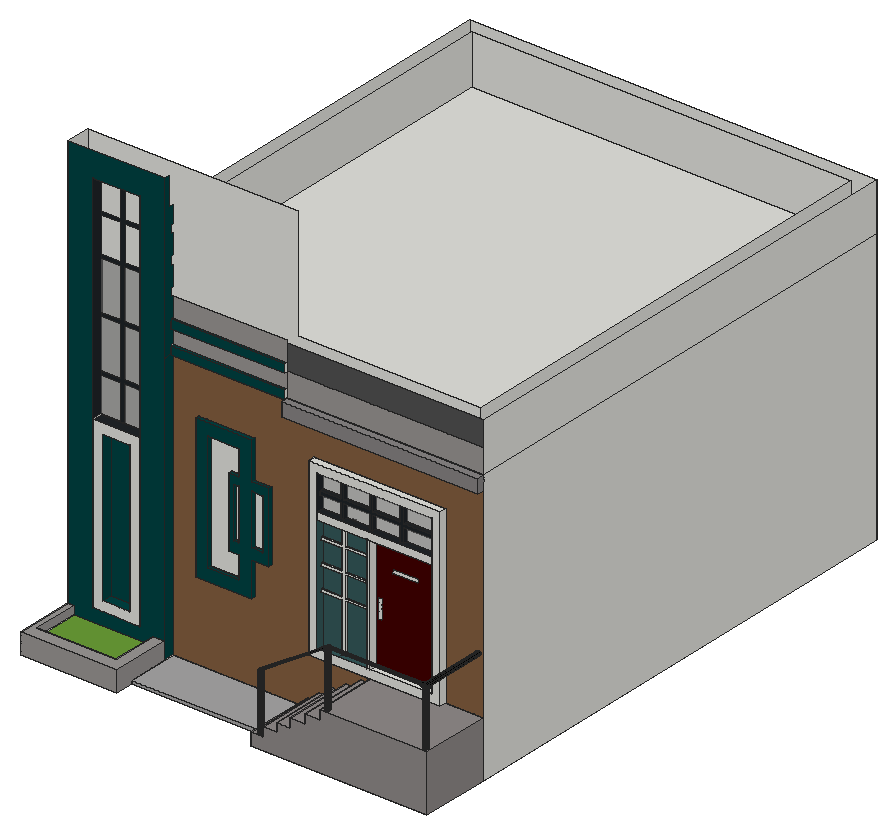
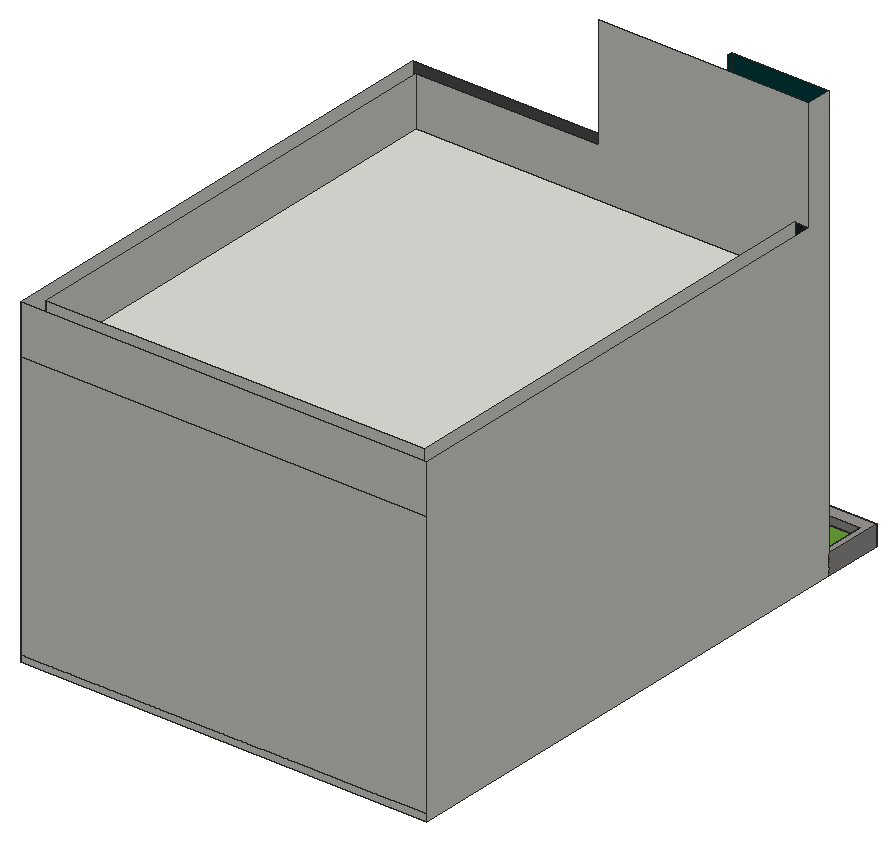
# SketchUp Ruby script. Lengths in inches.
U = 1.inch
M = Sketchup.active_model
def pt(a) = Geom::Point3d.new(a.map { |v| v * U })
def face(e, loops, mat)
  f = e.add_face(loops[0].map { |a| pt(a) })
  loops[1..].each { |l| e.add_face(l.map { |a| pt(a) }).erase! }
  f.material = f.back_material = mat if mat
  f
end
# faces: each face lists its corners as indices into pts; further lists are holes
def faces(e, pts, list, mat = nil) = list.each { |f| face(e, (f[0].is_a?(Array) ? f : [f]).map { |l| l.map { |i| pts[i] } }, mat) }
# xy, xz, yz: faces in a plane at the given z, y or x. An outline is a flat list of corners, or four numbers for a rectangle; further outlines are holes
def ring(l) = l.size == 4 ? [[l[0], l[1]], [l[2], l[1]], [l[2], l[3]], [l[0], l[3]]] : l.each_slice(2).to_a
def flat(e, list, mat, &to3) = list.each { |f| face(e, (f[0].is_a?(Array) ? f : [f]).map { |l| ring(l).map { |u, v| to3.(u, v) } }, mat) }
def xy(e, z, list, mat = nil) = flat(e, list, mat) { |x, y| [x, y, z] }
def xz(e, y, list, mat = nil) = flat(e, list, mat) { |x, z| [x, y, z] }
def yz(e, x, list, mat = nil) = flat(e, list, mat) { |y, z| [x, y, z] }
def lines(e, pts, list) = list.each { |a, b| e.add_line(pt(pts[a]), pt(pts[b])) }
# prism: a flat outline (further loops are holes) pulled along v
def prism(e, loops, v, mat = nil)
  f = face(e, loops, mat); d = Geom::Vector3d.new(v.map { |x| x * U })
  f.pushpull(f.normal.samedirection?(d) ? d.length : -d.length)
end
def box(e, o, s, mat = nil) = prism(e, [[o, [o[0] + s[0], o[1], o[2]], [o[0] + s[0], o[1] + s[1], o[2]], [o[0], o[1] + s[1], o[2]]]], [0, 0, s[2]], mat)
def at(x, y, z, deg = 0) = Geom::Transformation.translation(pt([x, y, z])) * Geom::Transformation.rotation(ORIGIN, Z_AXIS, deg.degrees)
def axes(o, x, y, z) = Geom::Transformation.new([*x, 0, *y, 0, *z, 0, *pt(o).to_a, 1])
def part(name) = M.definitions.add(name)
# library, detail: a bought-in or finely detailed component or shape, given as its bounding box
def library(name, o, s) = part(name).tap { |d| box(d.entities, o, s) }
def detail(e, o, s) = box(e.add_group.entities, o, s)
def put(e, d, t, mat = nil) = e.add_instance(d, t).tap { |i| i.material = mat if mat }
def group(e, t, mat = nil) = e.add_group.tap { |g| g.transformation = t; g.material = mat if mat }.entities
root = M.entities
M.materials.add("[0022_Maroon]").color = [66, 0, 0]
M.materials.add("[0079_Teal]").color = [0, 66, 66]
M.materials.add("[0081_CadetBlue]1").color = [52, 88, 89]
M.materials.add("[0099_LightSteelBlue]").color = [32, 36, 40]
M.materials.add("[0137_Black]").color = [0, 0, 0]
M.materials.add("[Brick Antique 01]").color = [132, 94, 64]
M.materials.add("[Brick Tumbled]").color = [135, 132, 132]
M.materials.add("[Concrete Aggregate Smoke]").color = [154, 150, 148]
M.materials.add("[Grass Dark Green]").color = [106, 157, 55]
M.materials.add("[Sketchy Scales]").color = [81, 81, 81]
M.materials.add("[Stone Marble]").color = [143, 138, 136]
M.materials.add("[Stone Vein Gray]").color = [166, 165, 165]
M.materials.add("[Translucent Glass Gray]").color = [128, 128, 128]
M.materials["[Translucent Glass Gray]"].alpha = 0.5
xy(root,0,[[0,0,0,51,5.305,51,5.305,11.375,72.805,11.375,72.805,51,82.708,51,82.708,0],[197.432,0,348,60],[5.305,11.375,72.805,51],[82.708,15.477,197.432,60],[0,51,82.708,60],
  [0,60,348,480]])
xy(root,3,[[82.708,15.477,197.432,60]],"[Stone Vein Gray]")
xy(root,10.4,[[202.157,1.901,201.64,1.969,201.157,2.169,200.743,2.487,200.425,2.901,200.225,3.383,200.157,3.901,200.225,4.419,200.425,4.901,200.743,5.315,201.157,5.633,201.64,5.833,202.157,5.901,202.675,5.833,203.157,5.633,203.571,5.315,203.889,4.901,204.089,4.419,204.157,3.901,204.089,3.383,203.889,2.901,203.571,2.487,203.157,2.169,202.675,1.969]],"[0137_Black]")
xy(root,10.4,[[[197.432,0,207.495,60],[202.157,1.901,201.64,1.969,201.157,2.169,200.743,2.487,200.425,2.901,200.225,3.383,200.157,3.901,200.225,4.419,200.425,4.901,200.743,5.315,201.157,5.633,201.64,5.833,202.157,5.901,202.675,5.833,203.157,5.633,203.571,5.315,203.889,4.901,204.089,4.419,204.157,3.901,204.089,3.383,203.889,2.901,203.571,2.487,203.157,2.169,202.675,1.969]]],"[Stone Marble]")
xy(root,10.6875,[[5.305,11.375,72.805,51]],"[Grass Dark Green]")
xy(root,17.625,[[0,0,82.708,0,82.708,51,72.805,51,72.805,11.375,5.305,11.375,5.305,51,0,51]],"[Concrete Aggregate Smoke]")
xy(root,18,[[207.495,0,219.245,60]],"[Stone Marble]")
xy(root,21.214,[[21.214,51,61.494,60]])
xy(root,25.5,[[219.245,0,230.745,60]],"[Stone Marble]")
xy(root,29.718,[[29.718,51,52.99,60]],"[0079_Teal]")
xy(root,33,[[230.745,0,243.245,60]],"[Stone Marble]")
xy(root,40.5,[[243.245,0,255.87,60]],"[Stone Marble]")
xy(root,48,[[343.717,1.809,343.199,1.877,342.717,2.077,342.303,2.395,341.985,2.809,341.785,3.292,341.717,3.809,341.785,4.327,341.985,4.809,342.303,5.223,342.717,5.541,343.199,5.741,343.717,5.809,344.235,5.741,344.717,5.541,345.131,5.223,345.449,4.809,345.649,4.327,345.717,3.809,345.649,3.292,345.449,2.809,345.131,2.395,344.717,2.077,344.235,1.877],[203.358,54,255.87,60],[255.87,54,315.483,60]])
xy(root,48,[[259.592,1.809,259.074,1.877,258.592,2.077,258.178,2.395,257.86,2.809,257.66,3.292,257.592,3.809,257.66,4.327,257.86,4.809,258.178,5.223,258.592,5.541,259.074,5.741,259.592,5.809,260.11,5.741,260.592,5.541,261.006,5.223,261.324,4.809,261.524,4.327,261.592,3.809,261.524,3.292,261.324,2.809,261.006,2.395,260.592,2.077,260.11,1.877]],"[0137_Black]")
xy(root,48,[[[255.87,0,348,0,348,60,315.483,60,315.483,54,255.87,54],[259.592,1.809,259.074,1.877,258.592,2.077,258.178,2.395,257.86,2.809,257.66,3.292,257.592,3.809,257.66,4.327,257.86,4.809,258.178,5.223,258.592,5.541,259.074,5.741,259.592,5.809,260.11,5.741,260.592,5.541,261.006,5.223,261.324,4.809,261.524,4.327,261.592,3.809,261.524,3.292,261.324,2.809,261.006,2.395,260.592,2.077,260.11,1.877],[343.717,1.809,343.199,1.877,342.717,2.077,342.303,2.395,341.985,2.809,341.785,3.292,341.717,3.809,341.785,4.327,341.985,4.809,342.303,5.223,342.717,5.541,343.199,5.741,343.717,5.809,344.235,5.741,344.717,5.541,345.131,5.223,345.449,4.809,345.649,4.327,345.717,3.809,345.649,3.292,345.449,2.809,345.131,2.395,344.717,2.077,344.235,1.877]]],"[Stone Marble]")
xy(root,54.949,[[252.87,54,255.87,60],[255.87,54,308.534,60],[228.307,58.5,231.307,60],[228.307,60,231.307,69.625]])
xy(root,54.949,[[210.307,54,228,60],[228,54,252.87,54,252.87,60,231.307,60,231.307,58.5,228.307,58.5,228.307,60,228,60]],"[0081_CadetBlue]1")
xy(root,57.305,[[202.157,1.901,202.675,1.969,203.157,2.169,203.571,2.487,203.889,2.901,204.089,3.383,204.157,3.901,204.089,4.419,203.889,4.901,203.571,5.315,203.157,5.633,202.675,5.833,202.157,5.901,201.64,5.833,201.157,5.633,200.743,5.315,200.425,4.901,200.225,4.419,200.157,3.901,200.225,3.383,200.425,2.901,200.743,2.487,201.157,2.169,201.64,1.969]],"[0137_Black]")
xy(root,71.632,[[104.425,57,152.3,60]],"[0079_Teal]")
xy(root,82.332,[[115.125,57,141.6,60]],"[0079_Teal]")
xy(root,94.905,[[259.592,1.809,260.11,1.877,260.592,2.077,261.006,2.395,261.324,2.809,261.524,3.292,261.592,3.809,261.524,4.327,261.324,4.809,261.006,5.223,260.592,5.541,260.11,5.741,259.592,5.809,259.074,5.741,258.592,5.541,258.178,5.223,257.86,4.809,257.66,4.327,257.592,3.809,257.66,3.292,257.86,2.809,258.178,2.395,258.592,2.077,259.074,1.877]],"[0137_Black]")
xy(root,96.949,[[210.307,58.5,228.307,60],[231.307,58.5,252.87,60],[210.307,60,228.307,69.625],[231.307,60,252.87,69.625]])
xy(root,98.949,[[210.307,58.5,228.307,60],[231.307,58.5,252.87,60],[210.307,60,228.307,69.625],[231.307,60,252.87,69.625]])
xy(root,101.329,[[141.6,57,152.3,60]])
xy(root,101.329,[[132.65,57,141.6,60],[152.3,57,166.837,60]],"[0079_Teal]")
xy(root,110.557,[[136.68,57,141.6,60],[152.3,57,161.992,60]],"[0079_Teal]")
xy(root,116.949,[[210.307,58.5,228.307,60],[231.307,58.5,252.87,60],[210.307,60,228.307,69.625],[231.307,60,252.87,69.625]])
xy(root,118.949,[[210.307,58.5,228.307,60],[231.307,58.5,252.87,60],[210.307,60,228.307,69.625],[231.307,60,252.87,69.625]])
xy(root,136.949,[[210.307,58.5,228.307,60],[231.307,58.5,252.87,60],[210.307,60,228.307,69.625],[231.307,60,252.87,69.625]])
xy(root,138.949,[[210.307,58.5,228.307,60],[231.307,58.5,252.87,60],[210.307,60,228.307,69.625],[231.307,60,252.87,69.625]])
xy(root,154.051,[[252.87,54,255.87,60],[255.87,54,308.534,60],[228.307,58.5,231.307,60],[228.307,60,231.307,69.625]])
xy(root,154.051,[[210.307,54,210.307,60,228.307,60,228.307,58.5,231.307,58.5,231.307,60,252.87,60,252.87,54]],"[0081_CadetBlue]1")
xy(root,154.307,[[136.68,57,141.6,60],[152.3,57,161.992,60]],"[0079_Teal]")
xy(root,157.286,[[29.718,51,52.99,60]],"[0079_Teal]")
xy(root,160.051,[[228.307,57,231.307,60],[252.87,57,255.87,60],[279.245,57,282.245,60]])
xy(root,160.051,[[210.307,54,308.534,54,308.534,60,282.245,60,282.245,57,279.245,57,279.245,60,255.87,60,255.87,57,252.87,57,252.87,60,231.307,60,231.307,57,228.307,57,228.307,60,210.307,60]],"[0099_LightSteelBlue]")
xy(root,161.454,[[132.65,57,141.6,60],[152.3,57,166.837,60]],"[0079_Teal]")
xy(root,165.791,[[21.214,51,61.494,60]],"[0099_LightSteelBlue]")
xy(root,172.051,[[210.307,57,228.307,60],[231.307,57,252.87,60],[255.87,57,279.245,60],[282.245,57,308.534,60]],"[0099_LightSteelBlue]")
xy(root,175.051,[[210.307,57,228.307,60],[231.307,57,252.87,60],[255.87,57,279.245,60],[282.245,57,308.534,60]],"[0099_LightSteelBlue]")
xy(root,183.119,[[115.125,57,141.6,60]],"[0079_Teal]")
xy(root,190.051,[[228.307,57,231.307,60],[252.87,57,255.87,60],[279.245,57,282.245,60]])
xy(root,190.051,[[210.307,54,210.307,60,228.307,60,228.307,57,231.307,57,231.307,60,252.87,60,252.87,57,255.87,57,255.87,60,279.245,60,279.245,57,282.245,57,282.245,60,308.534,60,308.534,54]],"[0099_LightSteelBlue]")
xy(root,193.82,[[104.425,57,152.3,60]],"[0079_Teal]")
xy(root,197,[[203.358,54,315.483,60]])
xy(root,222,[[180,54,348,60]],"[Brick Tumbled]")
xy(root,234,[[12,72,336,468]])
xy(root,234,[[82.708,57.5,180,60]],"[0081_CadetBlue]1")
xy(root,234,[[180,54,348,60]],"[Brick Tumbled]")
xy(root,241.06,[[82.708,57.5,180,60]],"[0079_Teal]")
xy(root,254.155,[[82.708,57.5,180,60]],"[0081_CadetBlue]1")
xy(root,261.216,[[82.708,57.5,180,60]],"[0079_Teal]")
xz(root,0,[[0,0,82.708,17.625]],"[Concrete Aggregate Smoke]")
xz(root,0,[[197.432,0,348,0,348,48,255.87,48,255.87,40.5,243.245,40.5,243.245,33,230.745,33,230.745,25.5,219.245,25.5,219.245,18,207.495,18,207.495,10.4,197.432,10.4]],"[Stone Marble]")
xz(root,11.375,[[5.305,0,72.805,10.6875]])
xz(root,11.375,[[5.305,10.6875,72.805,17.625]],"[Concrete Aggregate Smoke]")
xz(root,15.477,[[82.708,0,197.432,3]],"[Stone Vein Gray]")
xz(root,51,[[0,0,5.305,17.625],[5.305,0,72.805,10.6875],[72.805,0,82.708,17.625],[[21.214,21.214,61.494,165.791],[29.718,29.718,52.99,157.286]]])
xz(root,51,[[[5.305,10.6875,72.805,10.6875,72.805,17.625,82.708,17.625,82.708,372,0,372,0,17.625,5.305,17.625],[21.214,21.214,61.494,350.786]]],"[0079_Teal]")
xz(root,54,[[[203.358,48,315.483,197],[210.307,54.949,308.534,190.051]],[252.87,54.949,255.87,154.051],[210.307,154.051,308.534,160.051]])
xz(root,54,[[180,222,348,234]],"[Brick Tumbled]")
xz(root,57,[[[104.425,71.632,152.3,71.632,152.3,101.329,141.6,101.329,141.6,82.332,115.125,82.332,115.125,183.119,141.6,183.119,141.6,161.454,132.65,161.454,132.65,101.329,166.837,101.329,166.837,161.454,152.3,161.454,152.3,193.82,104.425,193.82],[152.3,110.557,161.992,154.307],[136.68,110.557,141.6,154.307]]],"[0079_Teal]")
xz(root,57,[[228.307,160.051,231.307,160.051,231.307,172.051,252.87,172.051,252.87,160.051,255.87,160.051,255.87,172.051,279.245,172.051,279.245,160.051,282.245,160.051,282.245,172.051,308.534,172.051,308.534,175.051,282.245,175.051,282.245,190.051,279.245,190.051,279.245,175.051,255.87,175.051,255.87,190.051,252.87,190.051,252.87,175.051,231.307,175.051,231.307,190.051,228.307,190.051,228.307,175.051,210.307,175.051,210.307,172.051,228.307,172.051]],"[0099_LightSteelBlue]")
xz(root,57.5,[[82.708,234,180,241.06],[82.708,254.155,180,261.216]],"[0079_Teal]")
xz(root,58.5,[[228.307,54.949,231.307,54.949,231.307,96.949,252.87,96.949,252.87,98.949,231.307,98.949,231.307,116.949,252.87,116.949,252.87,118.949,231.307,118.949,231.307,136.949,252.87,136.949,252.87,138.949,231.307,138.949,231.307,154.051,228.307,154.051,228.307,138.949,210.307,138.949,210.307,136.949,228.307,136.949,228.307,118.949,210.307,118.949,210.307,116.949,228.307,116.949,228.307,98.949,210.307,98.949,210.307,96.949,228.307,96.949]])
xz(root,60,[[82.708,0,197.432,3],[197.432,0,197.432,10.4,207.495,10.4,207.495,18,219.245,18,219.245,25.5,230.745,25.5,230.745,33,243.245,33,243.245,40.5,255.87,40.5,255.87,48,348,48,348,0],[[21.214,21.214,61.494,165.791],[29.718,29.718,52.99,157.286]],[[203.358,48,315.483,197],[210.307,54.949,308.534,190.051]],[252.87,54.949,255.87,154.051],
  [[104.425,71.632,104.425,193.82,152.3,193.82,152.3,161.454,166.837,161.454,166.837,101.329,132.65,101.329,132.65,161.454,141.6,161.454,141.6,183.119,115.125,183.119,115.125,82.332,141.6,82.332,141.6,101.329,152.3,101.329,152.3,71.632],[152.3,110.557,161.992,154.307],[136.68,110.557,141.6,154.307]],[115.125,82.332,141.6,82.332,141.6,101.329,132.65,101.329,132.65,161.454,141.6,161.454,141.6,183.119,115.125,183.119],[258.424,92.662,261.237,108.662],[136.68,110.557,141.6,154.307],[152.3,110.557,161.992,154.307],
  [270.914,131.531,292.789,134.718],[210.307,154.051,308.534,160.051],[228.307,160.051,228.307,172.051,210.307,172.051,210.307,175.051,228.307,175.051,228.307,190.051,231.307,190.051,231.307,175.051,252.87,175.051,252.87,190.051,255.87,190.051,255.87,175.051,279.245,175.051,279.245,190.051,282.245,190.051,282.245,175.051,308.534,175.051,308.534,172.051,282.245,172.051,282.245,160.051,279.245,160.051,279.245,172.051,255.87,172.051,255.87,160.051,252.87,160.051,252.87,172.051,231.307,172.051,231.307,160.051],[180,222,348,234]])
xz(root,60,[[[255.87,54.949,308.534,154.051],[270.914,131.531,292.789,134.718],[258.424,92.662,261.237,108.662]]],"[0022_Maroon]")
xz(root,60,[[29.718,29.718,52.99,157.286]],"[0079_Teal]")
xz(root,60,[[210.307,54.949,228.307,96.949],[231.307,54.949,252.87,96.949],[210.307,98.949,228.307,116.949],[231.307,98.949,252.87,116.949],[210.307,118.949,228.307,136.949],
  [231.307,118.949,252.87,136.949],[210.307,138.949,228.307,154.051],[231.307,138.949,252.87,154.051]],"[0081_CadetBlue]1")
xz(root,60,[[38.354,165.791,41.354,165.791,41.354,195.791,61.494,195.791,61.494,198.791,41.354,198.791,41.354,240.791,61.494,240.791,61.494,243.791,41.354,243.791,41.354,285.791,61.494,285.791,61.494,288.791,41.354,288.791,41.354,318.791,61.494,318.791,61.494,321.791,41.354,321.791,41.354,350.786,38.354,350.786,38.354,321.791,21.214,321.791,21.214,318.791,38.354,318.791,38.354,288.791,21.214,288.791,21.214,285.791,38.354,285.791,38.354,243.791,21.214,243.791,21.214,240.791,38.354,240.791,38.354,198.791,21.214,198.791,21.214,195.791,38.354,195.791]],"[0099_LightSteelBlue]")
xz(root,60,[[[82.708,3,197.432,3,197.432,10.4,207.495,10.4,207.495,18,219.245,18,219.245,25.5,230.745,25.5,230.745,33,243.245,33,243.245,40.5,255.87,40.5,255.87,48,203.358,48,203.358,197,315.483,197,315.483,48,348,48,348,222,180,222,180,234,82.708,234],[104.425,71.632,104.425,193.82,152.3,193.82,152.3,161.454,166.837,161.454,166.837,101.329,152.3,101.329,152.3,71.632],[343.717,94,343.199,94.068,342.717,94.268,342.303,94.586,341.985,95,341.785,95.482,341.717,96,341.785,96.518,341.985,97,342.303,97.414,342.717,97.732,343.199,97.932,343.717,98,344.235,97.932,344.717,97.732,345.131,97.414,345.449,97,345.649,96.518,345.717,96,345.649,95.482,345.449,95,345.131,94.586,344.717,94.268,344.235,94.068]]],"[Brick Antique 01]")
xz(root,60,[[180,234,348,255],[82.708,241.06,180,254.155],[82.708,261.216,180,278.155]],"[Concrete Aggregate Smoke]")
xz(root,60,[[180,255,348,276]],"[Sketchy Scales]")
xz(root,60,[[210.307,160.051,228.307,172.051],[231.307,160.051,252.87,172.051],[255.87,160.051,279.245,172.051],[282.245,160.051,308.534,172.051],[21.214,165.791,38.354,195.791],
  [41.354,165.791,61.494,195.791],[210.307,175.051,228.307,190.051],[231.307,175.051,252.87,190.051],[255.87,175.051,279.245,190.051],[282.245,175.051,308.534,190.051],
  [21.214,198.791,38.354,240.791],[41.354,198.791,61.494,240.791],[21.214,243.791,38.354,285.791],[41.354,243.791,61.494,285.791]],"[Translucent Glass Gray]")
xz(root,69.625,[[228.307,54.949,228.307,96.949,210.307,96.949,210.307,98.949,228.307,98.949,228.307,116.949,210.307,116.949,210.307,118.949,228.307,118.949,228.307,136.949,210.307,136.949,210.307,138.949,228.307,138.949,228.307,154.051,231.307,154.051,231.307,138.949,252.87,138.949,252.87,136.949,231.307,136.949,231.307,118.949,252.87,118.949,252.87,116.949,231.307,116.949,231.307,98.949,252.87,98.949,252.87,96.949,231.307,96.949,231.307,54.949]])
xz(root,72,[[12,234,12,276,0,276,0,372,180,372,180,276,336,276,336,234]])
xz(root,468,[[12,234,336,276]])
xz(root,480,[[0,0,348,6],[0,6,348,234],[0,234,348,276]])
yz(root,0,[[51,0,51,372,72,372,72,276,480,276,480,0]])
yz(root,0,[[0,0,51,17.625]],"[Concrete Aggregate Smoke]")
yz(root,5.305,[[11.375,0,51,10.6875]])
yz(root,5.305,[[11.375,10.6875,51,17.625]],"[Concrete Aggregate Smoke]")
yz(root,12,[[72,234,468,276]])
yz(root,21.214,[[51,21.214,60,165.791]])
yz(root,21.214,[[51,165.791,60,350.786]],"[0099_LightSteelBlue]")
yz(root,29.718,[[51,29.718,60,157.286]],"[0079_Teal]")
yz(root,52.99,[[51,29.718,60,48],[51,48,60,157.286]],"[0079_Teal]")
yz(root,61.494,[[51,21.214,60,48],[51,48,60,165.791]])
yz(root,61.494,[[51,165.791,60,350.786]],"[0099_LightSteelBlue]")
yz(root,72.805,[[11.375,0,51,10.6875]])
yz(root,72.805,[[11.375,10.6875,51,17.625]],"[Concrete Aggregate Smoke]")
yz(root,82.708,[[15.477,0,51,3],[51,0,60,3],[57.5,234,60,241.06],[57.5,254.155,60,261.216]])
yz(root,82.708,[[51,3,60,234],[51,234,57.5,234,57.5,241.06,60,241.06,60,254.155,57.5,254.155,57.5,261.216,60,261.216,60,278.155,57.5,278.155,57.5,285.216,60,285.216,60,302.155,57.5,302.155,57.5,309.216,60,309.216,60,326.155,57.5,326.155,57.5,333.216,60,333.216,60,348,55.5,348,55.5,372,51,372]],"[0079_Teal]")
yz(root,82.708,[[0,0,15.477,0,15.477,3,51,3,51,17.625,0,17.625]],"[Concrete Aggregate Smoke]")
yz(root,104.425,[[57,71.632,60,193.82]],"[0079_Teal]")
yz(root,115.125,[[57,82.332,60,183.119]],"[0079_Teal]")
yz(root,132.65,[[57,101.329,60,161.454]],"[0079_Teal]")
yz(root,136.68,[[57,110.557,60,154.307]],"[0079_Teal]")
yz(root,141.6,[[57,161.454,60,183.119]])
yz(root,141.6,[[57,82.332,60,101.329],[57,110.557,60,154.307]],"[0079_Teal]")
yz(root,152.3,[[57,71.632,60,101.329],[57,110.557,60,154.307],[57,161.454,60,193.82]],"[0079_Teal]")
yz(root,161.992,[[57,110.557,60,154.307]],"[0079_Teal]")
yz(root,166.837,[[57,101.329,60,161.454]],"[0079_Teal]")
yz(root,180,[[57.5,234,60,241.06],[57.5,254.155,60,261.216]])
yz(root,180,[[54,222,60,234]],"[Brick Tumbled]")
yz(root,197.432,[[15.477,0,60,3]])
yz(root,197.432,[[0,0,0,10.4,60,10.4,60,3,15.477,3,15.477,0]],"[Stone Marble]")
yz(root,203.358,[[54,48,60,197]])
yz(root,207.495,[[0,10.4,60,18]],"[Stone Marble]")
yz(root,210.307,[[58.5,96.949,60,98.949],[60,96.949,69.625,98.949],[58.5,116.949,60,118.949],[60,116.949,69.625,118.949],[58.5,136.949,60,138.949],
  [60,136.949,69.625,138.949],[54,154.051,60,160.051],[57,172.051,60,175.051]])
yz(root,210.307,[[54,54.949,60,54.949,60,96.949,58.5,96.949,58.5,98.949,60,98.949,60,116.949,58.5,116.949,58.5,118.949,60,118.949,60,136.949,58.5,136.949,58.5,138.949,60,138.949,60,154.051,54,154.051]],"[0081_CadetBlue]1")
yz(root,210.307,[[54,160.051,60,160.051,60,172.051,57,172.051,57,175.051,60,175.051,60,190.051,54,190.051]],"[0099_LightSteelBlue]")
yz(root,219.245,[[0,18,60,25.5]],"[Stone Marble]")
yz(root,228.307,[[58.5,54.949,60,96.949],[60,54.949,69.625,96.949],[58.5,98.949,60,116.949],[60,98.949,69.625,116.949],[58.5,118.949,60,136.949],
  [60,118.949,69.625,136.949],[58.5,138.949,60,154.051],[60,138.949,69.625,154.051]])
yz(root,228.307,[[57,160.051,60,172.051],[57,175.051,60,190.051]],"[0099_LightSteelBlue]")
yz(root,230.745,[[0,25.5,60,33]],"[Stone Marble]")
yz(root,231.307,[[58.5,54.949,60,96.949],[60,54.949,69.625,96.949],[58.5,98.949,60,116.949],[60,98.949,69.625,116.949],[58.5,118.949,60,136.949],
  [60,118.949,69.625,136.949],[58.5,138.949,60,154.051],[60,138.949,69.625,154.051]])
yz(root,231.307,[[57,160.051,60,172.051],[57,175.051,60,190.051]],"[0099_LightSteelBlue]")
yz(root,243.245,[[0,33,60,40.5]],"[Stone Marble]")
yz(root,252.87,[[58.5,96.949,60,98.949],[60,96.949,69.625,98.949],[58.5,116.949,60,118.949],[60,116.949,69.625,118.949],[58.5,136.949,60,138.949],
  [60,136.949,69.625,138.949]])
yz(root,252.87,[[54,54.949,60,96.949],[54,96.949,58.5,98.949],[54,98.949,60,116.949],[54,116.949,58.5,118.949],[54,118.949,60,136.949],
  [54,136.949,58.5,138.949],[54,138.949,60,154.051]],"[0081_CadetBlue]1")
yz(root,252.87,[[57,160.051,60,172.051],[57,175.051,60,190.051]],"[0099_LightSteelBlue]")
yz(root,255.87,[[54,54.949,60,154.051]])
yz(root,255.87,[[57,160.051,60,172.051],[57,175.051,60,190.051]],"[0099_LightSteelBlue]")
yz(root,255.87,[[0,40.5,60,48]],"[Stone Marble]")
yz(root,279.245,[[57,160.051,60,172.051],[57,175.051,60,190.051]],"[0099_LightSteelBlue]")
yz(root,282.245,[[57,160.051,60,172.051],[57,175.051,60,190.051]],"[0099_LightSteelBlue]")
yz(root,308.534,[[54,54.949,60,154.051],[54,154.051,60,160.051],[57,172.051,60,175.051]])
yz(root,308.534,[[54,160.051,54,190.051,60,190.051,60,175.051,57,175.051,57,172.051,60,172.051,60,160.051]],"[0099_LightSteelBlue]")
yz(root,315.483,[[54,48,60,197]])
yz(root,336,[[72,234,468,276]])
yz(root,341.717,[[3.809,95.084,3.809,96,4.904,96,4.905,96.003,4.867,96.24,4.757,96.461,4.582,96.65,4.355,96.795,4.091,96.886,3.807,96.917,3.524,96.885,3.26,96.792,3.033,96.646,2.859,96.456,2.751,96.235,2.714,95.997,2.752,95.76,2.862,95.539,3.036,95.35,3.263,95.205,3.528,95.114],[3.809,95.084,4.095,95.115,4.359,95.208,4.585,95.354,4.759,95.544,4.868,95.765,4.904,96,3.809,96]],"[0137_Black]")
yz(root,348,[[60,0,480,234],[60,234,480,276]])
yz(root,348,[[54,222,60,234]],"[Brick Tumbled]")
yz(root,348,[[0,0,60,48]],"[Stone Marble]")
p = [[201.64,1.969,10.4],[202.157,1.901,10.4],[202.157,1.901,57.305],[201.64,1.969,57.305],[202.675,1.969,10.4],[202.675,1.969,57.305],
  [201.157,2.169,10.4],[201.157,2.169,57.305],[203.157,2.169,10.4],[203.157,2.169,57.305],[200.743,2.487,10.4],[200.743,2.487,57.305],
  [203.571,2.487,10.4],[203.571,2.487,57.305],[200.425,2.901,10.4],[200.425,2.901,57.305],[203.889,2.901,10.4],[203.889,2.901,57.305],
  [200.225,3.383,10.4],[200.225,3.383,57.305],[204.089,3.383,10.4],[204.089,3.383,57.305],[200.157,3.901,10.4],[200.157,3.901,57.305],
  [204.157,3.901,10.4],[204.157,3.901,57.305],[200.225,4.419,10.4],[200.225,4.419,57.305],[204.089,4.419,10.4],[204.089,4.419,57.305],
  [200.425,4.901,10.4],[200.425,4.901,57.305],[203.889,4.901,10.4],[203.889,4.901,57.305],[200.743,5.315,10.4],[200.743,5.315,57.305],
  [203.571,5.315,10.4],[203.571,5.315,57.305],[201.157,5.633,10.4],[201.157,5.633,57.305],[203.157,5.633,10.4],[203.157,5.633,57.305],
  [201.64,5.833,10.4],[201.64,5.833,57.305],[202.675,5.833,10.4],[202.675,5.833,57.305],[202.157,5.901,10.4],[202.157,5.901,57.305],
  [259.074,1.877,48],[259.592,1.809,48],[259.592,1.809,94.905],[259.074,1.877,94.905],[260.11,1.877,48],[260.11,1.877,94.905],
  [343.199,1.877,48],[343.717,1.809,48],[343.717,1.809,98],[343.199,1.877,97.932],[344.235,1.877,48],[344.235,1.877,97.932],
  [258.592,2.077,48],[258.592,2.077,94.905],[260.592,2.077,48],[260.592,2.077,94.905],[342.717,2.077,48],[342.717,2.077,97.732],
  [344.717,2.077,48],[344.717,2.077,97.732],[258.178,2.395,48],[258.178,2.395,94.905],[261.006,2.395,48],[261.006,2.395,94.905],
  [342.303,2.395,48],[342.303,2.395,97.414],[345.131,2.395,48],[345.131,2.395,97.414],[257.86,2.809,48],[257.86,2.809,94.905],
  [261.324,2.809,48],[261.324,2.809,94.905],[341.985,2.809,48],[341.985,2.809,97],[345.449,2.809,48],[345.449,2.809,97],
  [257.66,3.292,48],[257.66,3.292,94.905],[261.524,3.292,48],[261.524,3.292,94.905],[341.785,3.292,48],[341.785,3.292,96.518],
  [345.649,3.292,48],[345.649,3.292,96.518],[257.592,3.809,48],[257.592,3.809,94.905],[261.592,3.809,48],[261.592,3.809,94.905],
  [341.717,3.809,48],[341.717,3.809,96],[341.717,3.809,95.084],[341.717,3.809,94.011],[345.717,3.809,48],[345.717,3.809,96],
  [257.66,4.327,48],[257.66,4.327,94.905],[261.524,4.327,48],[261.524,4.327,94.905],[341.771,4.218,94.043],[341.785,4.327,94.082],
  [341.785,4.327,48],[345.649,4.327,48],[345.649,4.327,95.482],[257.86,4.809,48],[257.86,4.809,94.905],[261.324,4.809,48],
  [261.324,4.809,94.905],[341.985,4.809,48],[341.785,4.327,95.482],[341.985,4.809,95],[345.449,4.809,48],[345.449,4.809,95],
  [258.178,5.223,48],[258.178,5.223,94.905],[261.006,5.223,48],[261.006,5.223,94.905],[342.303,5.223,48],[342.303,5.223,94.586],
  [345.131,5.223,48],[345.131,5.223,94.586],[258.592,5.541,48],[258.592,5.541,94.905],[260.592,5.541,48],[260.592,5.541,94.905],
  [342.717,5.541,48],[342.717,5.541,94.268],[344.717,5.541,48],[344.717,5.541,94.268],[259.074,5.741,48],[259.074,5.741,94.905],
  [260.11,5.741,48],[260.11,5.741,94.905],[343.199,5.741,48],[343.199,5.741,94.068],[344.235,5.741,48],[344.235,5.741,94.068],
  [259.592,5.809,48],[259.592,5.809,94.905],[343.717,5.809,48],[343.717,5.809,94],[202.592,4.45,57.737],[202.642,4.186,57.66],
  [202.659,3.9,57.633],[202.642,3.619,57.659],[202.592,3.355,57.735],[202.512,3.128,57.856],[202.408,2.953,58.014],[202.287,2.843,58.199],
  [202.157,2.806,58.397],[202.027,2.842,58.596],[201.906,2.951,58.781],[201.802,3.125,58.94],[201.722,3.352,59.063],[201.672,3.616,59.14],
  [201.655,3.899,59.167],[201.672,4.183,59.141],[201.722,4.447,59.065],[201.802,4.674,58.944],[201.906,4.849,58.786],[202.027,4.959,58.601],
  [202.157,4.997,58.403],[202.287,4.96,58.204],[202.408,4.851,58.019],[202.512,4.677,57.86],[259.592,3.809,94.905],[259.865,3.809,95.084],
  [259.856,3.528,95.114],[259.856,4.095,95.115],[259.829,3.263,95.205],[259.785,3.036,95.35],[259.829,4.359,95.208],[259.785,4.585,95.354],
  [259.729,2.862,95.539],[259.729,4.759,95.544],[259.663,2.752,95.76],[259.663,4.868,95.765],[259.592,2.714,95.997],[259.592,4.905,96.003],
  [259.462,2.751,96.196],[259.462,4.867,96.201],[259.341,2.86,96.381],[259.341,4.757,96.386],[259.237,3.033,96.54],[259.237,4.583,96.544],
  [259.157,3.26,96.663],[259.157,4.355,96.665],[259.107,3.524,96.74],[259.09,3.807,96.767],[259.107,4.091,96.741],[341.703,3.702,94.003],
  [341.636,3.193,94.099],[341.575,2.727,94.324],[341.523,2.333,94.664],[341.484,2.041,95.095],[341.462,1.869,95.587],[341.456,1.829,96.108],
  [341.469,1.924,96.621],[341.498,2.148,97.092],[341.543,2.485,97.489],[341.599,2.912,97.784],[341.663,3.4,97.957],[341.731,3.916,97.997],
  [341.798,4.425,97.901],[341.86,4.892,97.676],[341.911,5.285,97.336],[341.95,5.577,96.905],[341.972,5.749,96.413],[341.978,5.789,95.892],
  [341.965,5.694,95.379],[341.936,5.47,94.908],[341.891,5.134,94.511],[341.835,4.707,94.216],[343.199,60,94.068],[343.717,60,94],
  [344.235,60,94.068],[342.717,60,94.268],[344.717,60,94.268],[342.303,60,94.586],[345.131,60,94.586],[341.985,60,95],
  [345.449,60,95],[341.785,60,95.482],[345.649,60,95.482],[341.717,3.528,95.114],[341.717,3.263,95.205],[341.717,4.095,95.115],
  [341.717,4.359,95.208],[260.094,3.808,95.233],[260.077,4.095,95.26],[260.027,4.359,95.337],[259.947,4.585,95.46],[259.843,4.759,95.619],
  [259.722,4.868,95.804],[259.722,2.752,95.799],[259.843,2.861,95.614],[259.947,3.036,95.456],[260.027,3.263,95.335],[260.077,3.528,95.259],
  [341.717,3.036,95.35],[341.717,4.585,95.354],[341.717,2.862,95.539],[341.717,4.759,95.544],[341.717,2.752,95.76],[341.717,4.904,96],
  [341.717,60,96],[345.717,60,96],[341.717,4.868,95.765],[341.717,2.714,95.997],[341.717,4.905,96.003],[259.521,2.751,96.235],
  [341.717,2.751,96.235],[341.785,60,96.518],[345.649,60,96.518],[259.521,4.867,96.24],[341.717,4.867,96.24],[259.455,2.859,96.456],
  [341.717,2.859,96.456],[259.455,4.757,96.461],[341.717,4.757,96.461],[259.399,3.033,96.646],[259.399,4.582,96.65],[341.985,60,97],
  [345.449,60,97],[341.717,3.033,96.646],[259.355,3.26,96.792],[259.355,4.355,96.795],[341.717,4.582,96.65],[341.717,3.26,96.792],
  [341.717,4.355,96.795],[259.328,3.524,96.885],[259.319,3.807,96.917],[259.328,4.091,96.886],[341.717,3.524,96.885],[341.717,4.091,96.886],
  [341.717,3.807,96.917],[342.303,60,97.414],[345.131,60,97.414],[342.717,60,97.732],[344.717,60,97.732],[343.199,60,97.932],
  [344.235,60,97.932],[343.717,60,98],[343.717,3.809,48],[343.717,3.809,96],[343.717,60,96],[259.592,3.809,48],
  [259.592,3.809,96],[202.157,3.901,10.4],[202.157,3.901,57.305],[202.157,3.901,58.4]]
faces(root,p,[[0,1,2,3],[1,4,5,2],[6,0,3,7],[4,8,9,5],[10,6,7,11],[8,12,13,9],[14,10,11,15],[12,16,17,13],
  [18,14,15,19],[16,20,21,17],[22,18,19,23],[20,24,25,21],[26,22,23,27],[24,28,29,25],[30,26,27,31],[28,32,33,29],
  [34,30,31,35],[32,36,37,33],[38,34,35,39],[36,40,41,37],[42,38,39,43],[40,44,45,41],[46,42,43,47],[44,46,47,45],
  [48,49,50,51],[49,52,53,50],[54,55,56,57],[55,58,59,56],[60,48,51,61],[52,62,63,53],[64,54,57,65],[58,66,67,59],
  [68,60,61,69],[62,70,71,63],[72,64,65,73],[66,74,75,67],[76,68,69,77],[70,78,79,71],[80,72,73,81],[74,82,83,75],
  [84,76,77,85],[78,86,87,79],[88,80,81,89],[82,90,91,83],[92,84,85,93],[86,94,95,87],[96,88,89,97,98,99],[90,100,101,91],
  [102,92,93,103],[94,104,105,95],[96,99,106,107,108],[100,109,110,101],[111,102,103,112],[104,113,114,105],[115,108,107,116,117],[109,118,119,110],
  [120,111,112,121],[113,122,123,114],[124,115,117,125],[118,126,127,119],[128,120,121,129],[122,130,131,123],[132,124,125,133],[126,134,135,127],
  [136,128,129,137],[130,138,139,131],[140,132,133,141],[134,142,143,135],[144,136,137,145],[138,144,145,139],[146,140,141,147],[142,146,147,143],
  [148,149,150,151,152,153,154,155,156,157,158,159,160,161,162,163,164,165,166,167,168,169,170,171],[151,150,172,173,174],[150,149,175,173,172],[153,152,176,177],[152,151,174,176],[149,148,178,175],[148,171,179,178],[154,153,177,180],
  [171,170,181,179],[155,154,180,182],[170,169,183,181],[156,155,182,184],[169,168,185,183],[156,184,186,157],[167,187,185,168],[157,186,188,158],
  [166,189,187,167],[158,188,190,159],[165,191,189,166],[159,190,192,160],[164,193,191,165],[160,192,194,161],[161,194,195,162],[162,195,196,163],
  [163,196,193,164],[99,197,198,199,200,201,202,203,204,205,206,207,208,209,210,211,212,213,214,215,216,217,218,219,107,116,97,98],[116,107,106,99,98,97],[147,141,220,221],[143,147,221,222],[141,133,223,220],[135,143,222,224],[133,125,225,223],
  [127,135,224,226],[125,117,227,225],[119,127,226,228],[117,116,229,227],[110,119,228,230],[176,174,231,232],[174,173,98,231],[173,175,233,98],
  [175,178,234,233],[235,236,237,238,239,240,185,187,189,191,193,196,195,194,192,190,188,186,184,241,242,243,244,245],[177,176,232,246],[178,179,247,234],[180,177,246,248],[179,181,249,247],[182,180,248,250],[116,97,251,252,229],
  [101,110,230,253],[181,183,254,249],[184,182,250,255],[183,185,256,251,254],[257,184,255,258],[257,186,184],[97,89,259,252,251],[91,101,253,260],
  [185,261,262,256],[261,185,187],[263,188,186,257],[263,257,258,264],[261,187,189,265],[261,265,266,262],[267,190,188,263],[265,189,191,268],
  [89,81,269,259],[83,91,260,270],[267,263,264,271],[272,192,190,267],[268,191,193,273],[265,268,274,266],[272,267,271,275],[268,273,276,274],
  [277,194,192,272],[278,195,194,277],[279,196,195,278],[273,193,196,279],[277,272,275,280],[273,279,281,276],[278,277,280,282],[279,278,282,281],
  [81,73,283,269],[75,83,270,284],[73,65,285,283],[67,75,284,286],[65,57,287,285],[59,67,286,288],[57,56,289,287],[56,59,288,289]],"[0137_Black]")
lines(root,p,[[290,291],[291,292],[293,172],[294,97],[295,296],[297,294],[296,297],[97,291],[172,294]])
